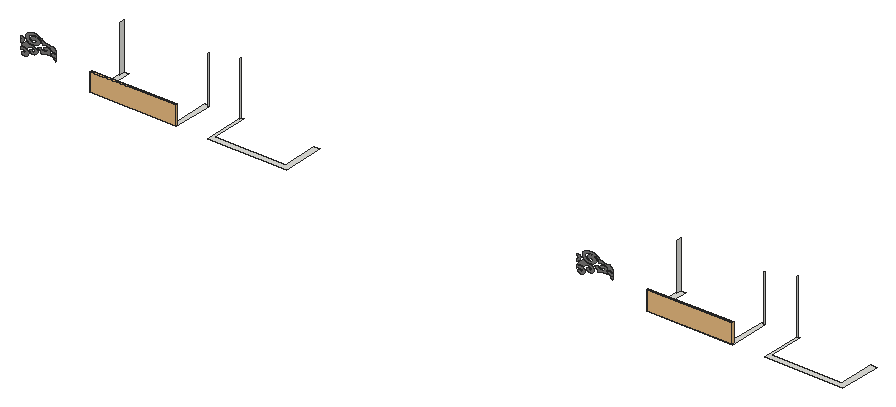
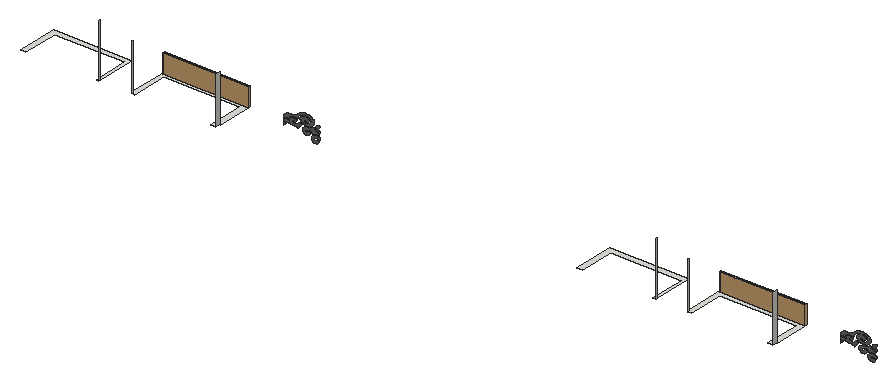
# SketchUp Ruby script. Lengths in inches.
U = 1.inch
M = Sketchup.active_model
def pt(a) = Geom::Point3d.new(a.map { |v| v * U })
def face(e, loops, mat)
  f = e.add_face(loops[0].map { |a| pt(a) })
  loops[1..].each { |l| e.add_face(l.map { |a| pt(a) }).erase! }
  f.material = f.back_material = mat if mat
  f
end
# faces: each face lists its corners as indices into pts; further lists are holes
def faces(e, pts, list, mat = nil) = list.each { |f| face(e, (f[0].is_a?(Array) ? f : [f]).map { |l| l.map { |i| pts[i] } }, mat) }
# xy, xz, yz: faces in a plane at the given z, y or x. An outline is a flat list of corners, or four numbers for a rectangle; further outlines are holes
def ring(l) = l.size == 4 ? [[l[0], l[1]], [l[2], l[1]], [l[2], l[3]], [l[0], l[3]]] : l.each_slice(2).to_a
def flat(e, list, mat, &to3) = list.each { |f| face(e, (f[0].is_a?(Array) ? f : [f]).map { |l| ring(l).map { |u, v| to3.(u, v) } }, mat) }
def xy(e, z, list, mat = nil) = flat(e, list, mat) { |x, y| [x, y, z] }
def xz(e, y, list, mat = nil) = flat(e, list, mat) { |x, z| [x, y, z] }
def yz(e, x, list, mat = nil) = flat(e, list, mat) { |y, z| [x, y, z] }
def lines(e, pts, list) = list.each { |a, b| e.add_line(pt(pts[a]), pt(pts[b])) }
# prism: a flat outline (further loops are holes) pulled along v
def prism(e, loops, v, mat = nil)
  f = face(e, loops, mat); d = Geom::Vector3d.new(v.map { |x| x * U })
  f.pushpull(f.normal.samedirection?(d) ? d.length : -d.length)
end
def box(e, o, s, mat = nil) = prism(e, [[o, [o[0] + s[0], o[1], o[2]], [o[0] + s[0], o[1] + s[1], o[2]], [o[0], o[1] + s[1], o[2]]]], [0, 0, s[2]], mat)
def at(x, y, z, deg = 0) = Geom::Transformation.translation(pt([x, y, z])) * Geom::Transformation.rotation(ORIGIN, Z_AXIS, deg.degrees)
def axes(o, x, y, z) = Geom::Transformation.new([*x, 0, *y, 0, *z, 0, *pt(o).to_a, 1])
def part(name) = M.definitions.add(name)
# library, detail: a bought-in or finely detailed component or shape, given as its bounding box
def library(name, o, s) = part(name).tap { |d| box(d.entities, o, s) }
def detail(e, o, s) = box(e.add_group.entities, o, s)
def put(e, d, t, mat = nil) = e.add_instance(d, t).tap { |i| i.material = mat if mat }
def group(e, t, mat = nil) = e.add_group.tap { |g| g.transformation = t; g.material = mat if mat }.entities
root = M.entities
M.materials.add("[0043_SaddleBrown]4").color = [124, 123, 122]
c1 = library("Glass Railing",[0,0,0],[139.5,4.76,42])
xy(root,541.1875,[[3051.26,558.125,3245.44,558.125,3245.44,647.91,3243.69,647.91,3243.69,651.03,3235.84,651.03,3235.84,570.83,3064.33,570.83,3064.33,651.03,3053.01,651.03,3053.01,640.11,3051.26,640.11],[3315.93,558.125,3493.19,558.125,3493.19,651.03,3480.11,651.03,3480.11,570.83,3322.22,570.83,3322.22,651.03,3315.93,651.03],[4301.88,558.125,4496.07,558.125,4496.07,647.91,4494.32,647.91,4494.32,651.03,4486.46,651.03,4486.46,570.83,4314.96,570.83,4314.96,651.03,4303.63,651.03,4303.63,640.11,4301.88,640.11],[4566.56,558.125,4743.81,558.125,4743.81,651.03,4730.74,651.03,4730.74,570.83,4572.84,570.83,4572.84,651.03,4566.56,651.03]])
xz(root,589.17,[[2879.79,541.67,2878.5,541.71,2877.26,541.9,2876.09,542.23,2875.05,542.69,2874.17,543.27,2873.48,543.93,2873,544.67,2872.76,545.44,2872.67,545.74,2872.68,546.04,2872.78,546.34,2872.97,546.62,2873.25,546.875,2873.6,547.09,2874.02,547.26,2874.48,547.37,2874.96,547.43,2875.46,547.43,2875.94,547.37,2876.4,547.25,2876.67,547.03,2876.96,546.83,2877.27,546.64,2877.59,546.45,2877.94,546.29,2878.3,546.13,2878.68,545.99,2879.07,545.87,2879.48,545.76,2879.89,545.66,2880.3125,545.58,2880.74,545.52,2881.31,545.82,2881.8,546.16,2882.23,546.53,2882.58,546.93,2882.85,547.36,2883.03,547.8,2883.13,548.25,2883.13,548.71,2883.04,549.16,2882.86,549.6,2882.6,550.03,2882.25,550.43,2881.52,551.04,2880.63,551.56,2879.62,551.98,2878.5,552.29,2877.3125,552.48,2876.09,552.55,2874.87,552.48,2873.68,552.29,2872.5625,551.98,2871.55,551.56,2870.66,551.04,2869.93,550.43,2869.93,554.9,2870.81,555.28,2871.74,555.61,2872.72,555.89,2873.74,556.1,2874.79,556.26,2875.85,556.35,2876.93,556.37,2878,556.33,2879.07,556.23,2880.11,556.07,2881.12,555.84,2882.09,555.55,2883.79,554.88,2885.29,554.04,2886.55,553.07,2887.54,551.99,2888.24,550.82,2888.62,549.61,2888.68,548.36,2888.42,547.13,2887.84,545.94,2886.95,544.83,2885.79,543.8125,2884.375,542.92,2883.4,542.41,2882.28,542.02,2881.06,541.77],[4130.41,541.67,4129.13,541.71,4127.88,541.9,4126.72,542.23,4125.67,542.69,4124.79,543.27,4124.1,543.93,4123.625,544.67,4123.39,545.44,4123.3,545.74,4123.3,546.04,4123.4,546.34,4123.6,546.62,4123.875,546.875,4124.23,547.09,4124.64,547.26,4125.1,547.37,4125.59,547.43,4126.08,547.43,4126.57,547.37,4127.03,547.25,4127.29,547.03,4127.58,546.83,4127.89,546.64,4128.22,546.45,4128.57,546.29,4128.93,546.13,4129.31,545.99,4129.7,545.87,4130.1,545.76,4130.51,545.66,4130.9375,545.58,4131.37,545.52,4131.93,545.82,4132.43,546.16,4132.86,546.53,4133.21,546.93,4133.48,547.36,4133.66,547.8,4133.75,548.25,4133.75,548.71,4133.66,549.16,4133.49,549.6,4133.22,550.03,4132.87,550.43,4132.14,551.04,4131.26,551.56,4130.24,551.98,4129.125,552.29,4127.9375,552.48,4126.71,552.55,4125.49,552.48,4124.3,552.29,4123.1875,551.98,4122.17,551.56,4121.29,551.04,4120.56,550.43,4120.56,554.9,4121.43,555.28,4122.36,555.61,4123.34,555.89,4124.36,556.1,4125.41,556.26,4126.48,556.35,4127.55,556.37,4128.63,556.33,4129.69,556.23,4130.74,556.07,4131.75,555.84,4132.72,555.55,4134.41,554.88,4135.91,554.04,4137.17,553.07,4138.16,551.99,4138.86,550.82,4139.24,549.61,4139.31,548.36,4139.04,547.13,4138.46,545.94,4137.58,544.83,4136.41,543.8125,4135,542.92,4134.02,542.41,4132.9,542.02,4131.68,541.77],[2899.8,551.33,2898.2,551.39,2896.65,551.65,2895.22,552.1,2893.98,552.73,2892.98,553.5,2892.27,554.38,2891.87,555.34,2891.8125,556.33,2891.875,556.63,2891.99,556.93,2892.15,557.23,2892.36,557.51,2892.62,557.77,2892.92,558.02,2893.25,558.25,2893.63,558.46,2894.04,558.64,2894.48,558.79,2894.94,558.92,2895.41,559.01,2895.5,558.58,2895.62,558.15,2895.78,557.72,2895.99,557.3,2896.23,556.89,2896.51,556.49,2896.83,556.1,2897.18,555.72,2897.58,555.35,2898,555,2898.46,554.67,2898.95,554.35,2899.88,554.64,2900.73,555.01,2901.48,555.46,2902.11,555.97,2902.6,556.54,2902.9375,557.15,2903.125,557.78,2903.15,558.42,2903.01,559.06,2902.72,559.68,2902.27,560.26,2901.6875,560.79,2900.85,561.59,2899.78,562.28,2898.53,562.84,2897.125,563.25,2895.62,563.49,2894.07,563.5625,2892.53,563.45,2891.05,563.17,2889.68,562.72,2888.46,562.13,2887.45,561.41,2886.67,560.59,2886.45,560.37,2886.25,560.14,2886.06,559.91,2885.88,559.68,2885.71,559.45,2885.56,559.21,2885.42,558.97,2885.29,558.72,2885.17,558.47,2885.07,558.23,2884.98,557.97,2884.91,557.72,2884.22,558.29,2883.41,558.79,2882.52,559.24,2881.54,559.61,2880.49,559.9,2879.39,560.11,2878.26,560.23,2877.11,560.27,2875.97,560.22,2874.84,560.08,2873.75,559.86,2872.71,559.56,2872.92,559.82,2873.12,560.09,2873.28,560.37,2873.42,560.65,2873.54,560.94,2873.62,561.23,2873.68,561.53,2873.71,561.82,2873.72,562.12,2873.69,562.41,2873.64,562.71,2873.5625,563,2874.7,563.53,2875.8,564.1,2876.86,564.7,2877.86,565.33,2878.81,565.99,2879.72,566.67,2880.5625,567.39,2881.36,568.12,2882.09,568.88,2882.76,569.66,2883.37,570.46,2883.92,571.27,2884.53,570.61,2885.24,569.98,2886.0625,569.4,2886.97,568.88,2887.96,568.41,2889.02,568.01,2890.14,567.68,2891.3125,567.42,2892.52,567.24,2893.76,567.13,2895,567.1,2896.24,567.14,2898.66,566.8,2900.95,566.2,2903.02,565.37,2904.83,564.32,2906.32,563.1,2907.4375,561.74,2908.15,560.28,2908.4375,558.77,2908.29,557.24,2907.71,555.76,2906.73,554.36,2905.36,553.09,2904.23,552.39,2902.89,551.85,2901.39,551.49],[4150.43,551.33,4148.82,551.39,4147.27,551.65,4145.84,552.1,4144.6,552.73,4143.6,553.5,4142.89,554.38,4142.5,555.34,4142.4375,556.33,4142.5,556.63,4142.61,556.93,4142.77,557.23,4142.98,557.51,4143.24,557.77,4143.54,558.02,4143.88,558.25,4144.26,558.46,4144.66,558.64,4145.1,558.79,4145.56,558.92,4146.04,559.01,4146.12,558.58,4146.24,558.15,4146.41,557.72,4146.61,557.3,4146.85,556.89,4147.14,556.49,4147.45,556.1,4147.81,555.72,4148.2,555.35,4148.625,555,4149.08,554.67,4149.57,554.35,4150.51,554.64,4151.36,555.01,4152.11,555.46,4152.73,555.97,4153.22,556.54,4153.5625,557.15,4153.75,557.78,4153.77,558.42,4153.64,559.06,4153.34,559.68,4152.9,560.26,4152.3125,560.79,4151.47,561.59,4150.41,562.28,4149.15,562.84,4147.75,563.25,4146.25,563.49,4144.7,563.5625,4143.16,563.45,4141.68,563.17,4140.3,562.72,4139.09,562.13,4138.07,561.41,4137.29,560.59,4137.08,560.37,4136.87,560.14,4136.68,559.91,4136.5,559.68,4136.34,559.45,4136.18,559.21,4136.04,558.97,4135.91,558.72,4135.8,558.47,4135.7,558.23,4135.61,557.97,4135.53,557.72,4134.84,558.29,4134.04,558.79,4133.14,559.24,4132.16,559.61,4131.12,559.9,4130.02,560.11,4128.89,560.23,4127.74,560.27,4126.59,560.22,4125.46,560.08,4124.37,559.86,4123.33,559.56,4123.55,559.82,4123.74,560.09,4123.91,560.37,4124.05,560.65,4124.16,560.94,4124.25,561.23,4124.31,561.53,4124.34,561.82,4124.34,562.12,4124.32,562.41,4124.27,562.71,4124.1875,563,4125.33,563.53,4126.43,564.1,4127.48,564.7,4128.49,565.33,4129.44,565.99,4130.34,566.67,4131.1875,567.39,4131.98,568.12,4132.71,568.88,4133.39,569.66,4134,570.46,4134.54,571.27,4135.15,570.61,4135.87,569.98,4136.6875,569.4,4137.59,568.88,4138.58,568.41,4139.65,568.01,4140.77,567.68,4141.9375,567.42,4143.15,567.24,4144.38,567.13,4145.625,567.1,4146.87,567.14,4149.29,566.8,4151.57,566.2,4153.65,565.37,4155.46,564.32,4156.94,563.1,4158.0625,561.74,4158.77,560.28,4159.0625,558.77,4158.92,557.24,4158.34,555.76,4157.35,554.36,4155.98,553.09,4154.85,552.39,4153.51,551.85,4152.01,551.49],[2950.32,553.96,2950.04,554.34,2949.75,554.71,2949.45,555.08,2949.13,555.4375,2948.8,555.8,2948.46,556.15,2948.11,556.5,2947.75,556.85,2947.37,557.19,2946.98,557.53,2946.59,557.86,2946.18,558.1875,2946.45,558.35,2946.75,558.5,2947.06,558.64,2947.38,558.76,2947.72,558.86,2948.08,558.95,2948.4375,559.03,2948.81,559.09,2949.18,559.13,2949.5625,559.15,2949.94,559.16,2950.32,559.15],
  [4200.95,553.96,4200.67,554.34,4200.375,554.71,4200.07,555.08,4199.76,555.4375,4199.43,555.8,4199.09,556.15,4198.37,556.85,4198,557.19,4197.61,557.53,4197.21,557.86,4196.8,558.1875,4197.08,558.35,4197.37,558.5,4197.68,558.64,4198.01,558.76,4198.35,558.86,4198.7,558.95,4199.0625,559.03,4199.43,559.09,4199.81,559.13,4200.1875,559.15,4200.57,559.16,4200.95,559.15],[2917.28,558.48,2917.16,559.39,2916.93,560.29,2916.59,561.18,2916.15,562.05,2915.6,562.9,2914.94,563.72,2914.19,564.51,2913.35,565.26,2912.41,565.97,2911.4,566.63,2910.3,567.25,2909.13,567.8125,2909.75,567.99,2910.36,568.17,2910.97,568.36,2911.57,568.55,2912.75,568.97,2913.33,569.18,2913.9,569.41,2914.46,569.64,2915.02,569.88,2915.57,570.125,2916.11,570.38,2916.21,569.18,2916.74,568.03,2917.66,566.98,2918.93,566.07,2920.5,565.36,2922.27,564.87,2924.18,564.625,2926.13,564.65,2928.02,564.93,2929.77,565.45,2931.3,566.2,2932.52,567.13,2932.55,567.42,2932.57,567.71,2932.58,568,2932.57,568.29,2932.55,568.58,2932.51,568.87,2932.46,569.16,2932.4,569.45,2932.32,569.73,2932.23,570.02,2932.12,570.3,2932,570.58,2931.41,570.74,2930.78,570.84,2930.13,570.875,2929.49,570.85,2928.86,570.76,2928.26,570.61,2927.7,570.4,2927.21,570.14,2926.79,569.84,2926.45,569.5,2926.21,569.13,2926.07,568.74,2925.66,568.85,2925.27,568.97,2924.89,569.11,2924.52,569.26,2924.18,569.43,2923.84,569.61,2923.53,569.8,2923.24,570,2922.97,570.22,2922.72,570.44,2922.5,570.68,2922.3,570.92,2922.89,571.87,2923.78,572.73,2924.9375,573.46,2926.3125,574.03,2927.85,574.42,2929.49,574.6,2931.15,574.58,2932.76,574.35,2934.27,573.91,2935.6,573.3,2936.7,572.54,2937.52,571.65,2936.96,570.85,2936.51,570.02,2936.1875,569.17,2935.99,568.3125,2935.91,567.44,2935.96,566.57,2936.14,565.7,2936.4375,564.85,2936.86,564.02,2937.4,563.21,2938.06,562.4375,2938.82,561.7,2936.94,561.8,2935.06,561.83,2933.17,561.79,2931.29,561.68,2929.43,561.51,2927.59,561.27,2925.77,560.96,2923.98,560.59,2922.23,560.15,2920.53,559.66,2918.88,559.1],[4167.91,558.48,4167.79,559.39,4167.56,560.29,4167.22,561.18,4166.77,562.05,4166.22,562.9,4165.57,563.72,4164.82,564.51,4163.97,565.26,4163.04,565.97,4162.02,566.63,4160.92,567.25,4159.76,567.8125,4160.375,567.99,4160.99,568.17,4162.19,568.55,4163.37,568.97,4163.95,569.18,4165.09,569.64,4165.64,569.88,4166.19,570.125,4166.73,570.38,4166.84,569.18,4167.36,568.03,4168.29,566.98,4169.56,566.07,4171.12,565.36,4172.9,564.87,4174.81,564.625,4176.75,564.65,4178.65,564.93,4180.4,565.45,4181.92,566.2,4183.14,567.13,4183.18,567.42,4183.2,567.71,4183.21,568,4183.2,568.29,4183.18,568.58,4183.14,568.87,4183.09,569.16,4183.03,569.45,4182.95,569.73,4182.85,570.02,4182.75,570.3,4182.63,570.58,4182.03,570.74,4181.41,570.84,4180.76,570.875,4180.11,570.85,4179.48,570.76,4178.88,570.61,4178.33,570.4,4177.84,570.14,4177.42,569.84,4177.08,569.5,4176.84,569.13,4176.69,568.74,4176.29,568.85,4175.89,568.97,4175.51,569.11,4175.15,569.26,4174.8,569.43,4174.47,569.61,4174.16,569.8,4173.87,570,4173.6,570.22,4173.35,570.44,4173.125,570.68,4172.92,570.92,4173.51,571.87,4174.4,572.73,4175.5625,573.46,4176.9375,574.03,4178.48,574.42,4180.11,574.6,4181.77,574.58,4183.39,574.35,4184.89,573.91,4186.23,573.3,4187.32,572.54,4188.15,571.65,4187.58,570.85,4187.14,570.02,4186.8125,569.17,4186.61,568.3125,4186.54,567.44,4186.59,566.57,4186.76,565.7,4187.0625,564.85,4187.49,564.02,4188.03,563.21,4188.68,562.4375,4189.45,561.7,4187.57,561.8,4185.68,561.83,4183.8,561.79,4181.92,561.68,4180.06,561.51,4178.21,561.27,4176.39,560.96,4174.61,560.59,4172.86,560.15,4171.16,559.66,4169.5,559.1],[2946.1,561.42,2945.01,561.51,2943.94,561.71,2942.95,562.01,2942.04,562.41,2941.25,562.89,2940.6,563.4375,2940.09,564.04,2939.75,564.69,2939.49,564.99,2939.33,565.31,2939.28,565.64,2939.33,565.97,2939.48,566.29,2939.74,566.59,2940.07,566.85,2940.49,567.07,2940.97,567.23,2941.48,567.33,2942.02,567.375,2942.57,567.35,2943.03,567.29,2943.48,567.21,2943.92,567.1,2944.34,566.96,2944.74,566.81,2945.12,566.63,2945.46,566.43,2945.78,566.22,2946.07,565.98,2946.32,565.74,2946.54,565.48,2946.71,565.21,2947.06,565.32,2947.4,565.45,2947.73,565.58,2948.05,565.71,2948.37,565.86,2948.97,566.16,2949.26,566.33,2949.54,566.5,2949.8125,566.67,2950.07,566.85,2950.32,567.04,2950.32,562.11,2949.35,561.78,2948.3,561.56,2947.21,561.43],[4196.73,561.42,4195.63,561.51,4194.57,561.71,4193.57,562.01,4192.67,562.41,4191.88,562.89,4191.22,563.4375,4190.71,564.04,4190.37,564.69,4190.12,564.99,4189.96,565.31,4189.9,565.64,4189.95,565.97,4190.11,566.29,4190.36,566.59,4190.7,566.85,4191.12,567.07,4191.59,567.23,4192.11,567.33,4192.65,567.375,4193.19,567.35,4193.66,567.29,4194.11,567.21,4194.55,567.1,4194.97,566.96,4195.37,566.81,4195.74,566.63,4196.09,566.43,4196.41,566.22,4196.69,565.98,4196.95,565.74,4197.16,565.48,4197.34,565.21,4197.68,565.32,4198.02,565.45,4198.68,565.71,4199.3,566.01,4199.6,566.16,4199.89,566.33,4200.17,566.5,4200.4375,566.67,4200.7,566.85,4200.95,567.04,4200.95,562.11,4199.97,561.78,4198.93,561.56,4197.84,561.43],
  [2869.93,564.47,2869.93,568.51,2871.02,568.79,2871.98,569.2,2872.78,569.74,2873.38,570.36,2873.75,571.04,2873.875,571.76,2873.75,572.48,2873.38,573.17,2872.78,573.79,2871.98,574.32,2871.02,574.73,2869.93,575.01,2869.93,578.44,2871.18,578.38,2872.4,578.2,2873.5625,577.92,2874.64,577.52,2875.61,577.03,2876.44,576.46,2877.125,575.8125,2877.64,575.11,2877.98,574.37,2878.13,573.61,2878.1,572.84,2877.87,572.08,2877.52,571.34,2877.11,570.62,2876.64,569.91,2876.1,569.22,2875.52,568.55,2874.87,567.89,2874.17,567.26,2873.42,566.65,2872.62,566.0625,2871.77,565.5,2870.87,564.97],[4120.56,564.47,4120.56,568.51,4121.64,568.79,4122.61,569.2,4123.4,569.74,4124,570.36,4124.375,571.04,4124.5,571.76,4124.375,572.48,4124,573.17,4123.4,573.79,4122.61,574.32,4121.64,574.73,4120.56,575.01,4120.56,578.44,4121.81,578.38,4123.03,578.2,4124.1875,577.92,4125.26,577.52,4126.23,577.03,4127.07,576.46,4127.75,575.8125,4128.27,575.11,4128.61,574.37,4128.76,573.61,4128.72,572.84,4128.49,572.08,4128.14,571.34,4127.73,570.62,4127.26,569.91,4126.73,569.22,4126.14,568.55,4125.5,567.89,4124.8,567.26,4124.05,566.65,4123.24,566.0625,4122.39,565.5,4121.5,564.97],[2950.32,568.52,2949.96,569.11,2949.46,569.67,2948.84,570.17,2948.11,570.62,2947.29,571,2946.38,571.3125,2945.42,571.54,2944.41,571.68,2943.38,571.73,2942.35,571.69,2941.34,571.57,2940.37,571.36,2939.92,572.72,2939.11,574.02,2937.94,575.22,2936.47,576.27,2934.72,577.15,2932.75,577.84,2930.62,578.31,2928.38,578.55,2926.12,578.55,2923.89,578.32,2921.75,577.85,2919.78,577.17,2919.72,578.89,2919.25,580.59,2918.39,582.23,2917.14,583.77,2915.55,585.19,2913.64,586.45,2911.45,587.53,2909.04,588.4,2906.4375,589.05,2903.71,589.45,2900.92,589.61,2898.12,589.52,2895.67,588.91,2893.45,588.01,2891.56,586.87,2890.07,585.52,2889.02,584.03,2888.47,582.4375,2888.43,580.81,2888.89,579.21,2889.86,577.6875,2891.28,576.31,2893.11,575.14,2895.27,574.19,2896.66,573.82,2898.16,573.62,2899.68,573.61,2901.18,573.8,2902.58,574.17,2903.83,574.7,2904.875,575.38,2905.67,576.18,2906.1875,577.0625,2906.4,577.99,2906.3,578.93,2905.9,579.83,2905.62,580.16,2905.24,580.45,2904.78,580.69,2904.25,580.87,2903.67,580.98,2903.06,581.02,2902.46,580.98,2901.88,580.87,2901.35,580.69,2900.89,580.45,2900.51,580.16,2900.23,579.83,2900.09,579.64,2899.93,579.45,2899.75,579.28,2899.54,579.11,2899.31,578.95,2899.06,578.8125,2898.79,578.68,2898.5,578.57,2898.2,578.46,2897.89,578.38,2897.57,578.31,2897.24,578.25,2896.66,578.46,2896.125,578.72,2895.64,579.01,2895.22,579.33,2894.87,579.69,2894.59,580.0625,2894.39,580.46,2894.27,580.87,2894.23,581.28,2894.27,581.69,2894.4,582.1,2894.61,582.49,2895,583.02,2895.48,583.52,2896.04,583.99,2896.68,584.42,2897.4,584.8,2898.17,585.13,2899,585.41,2899.88,585.63,2900.79,585.8,2901.72,585.9,2902.66,585.94,2903.61,585.92,2905.1,585.78,2906.55,585.51,2907.92,585.13,2909.2,584.64,2910.37,584.05,2911.39,583.36,2912.26,582.6,2912.95,581.78,2913.46,580.91,2913.78,580,2913.9,579.08,2913.81,578.15,2913.2,576.76,2912.28,575.43,2911.0625,574.2,2909.57,573.09,2907.84,572.12,2905.89,571.31,2903.79,570.67,2901.55,570.23,2899.24,569.99,2896.89,569.95,2894.5625,570.11,2892.29,570.48,2890.1,571.41,2888.12,572.5,2886.38,573.73,2884.92,575.1,2883.76,576.57,2882.92,578.12,2882.42,579.73,2882.26,581.36,2882.4375,582.99,2882.96,584.59,2883.82,586.14,2884.99,587.6,2886.8,589.2,2889.02,590.58,2891.59,591.72,2894.43,592.57,2897.46,593.12,2900.61,593.34,2903.77,593.23,2906.85,592.8,2909.77,592.05,2912.44,591.01,2914.79,589.71,2916.75,588.1875,2917.29,587.55,2917.88,586.9375,2918.52,586.34,2919.2,585.76,2919.92,585.2,2920.69,584.66,2921.5,584.14,2922.35,583.65,2923.23,583.1875,2924.15,582.75,2925.1,582.33,2926.08,581.95,2927.38,581.57,2928.72,581.23,2930.08,580.94,2931.47,580.7,2932.875,580.5,2934.3,580.36,2935.73,580.26,2937.17,580.2,2938.61,580.2,2940.05,580.25,2941.48,580.34,2942.91,580.49,2943.46,579.94,2944.03,579.4,2944.61,578.86,2945.2,578.33,2945.8,577.81,2946.42,577.28,2947.04,576.77,2948.32,575.75,2948.98,575.25,2949.65,574.75,2950.32,574.26],[4200.95,568.52,4200.58,569.11,4200.08,569.67,4199.46,570.17,4198.74,570.62,4197.91,571,4197.01,571.3125,4196.04,571.54,4195.04,571.68,4194.01,571.73,4192.98,571.69,4191.97,571.57,4190.99,571.36,4190.55,572.72,4189.73,574.02,4188.57,575.22,4187.09,576.27,4185.34,577.15,4183.37,577.84,4181.24,578.31,4179.01,578.55,4176.74,578.55,4174.51,578.32,4172.38,577.85,4170.4,577.17,4170.34,578.89,4169.875,580.59,4169.01,582.23,4167.77,583.77,4166.18,585.19,4164.27,586.45,4162.08,587.53,4159.66,588.4,4157.0625,589.05,4154.34,589.45,4151.55,589.61,4148.75,589.52,4146.29,588.91,4144.08,588.01,4142.19,586.87,4140.69,585.52,4139.65,584.03,4139.09,582.4375,4139.05,580.81,4139.52,579.21,4140.48,577.6875,4141.9,576.31,4143.73,575.14,4145.89,574.19,4147.29,573.82,4148.78,573.62,4150.31,573.61,4151.8,573.8,4153.2,574.17,4154.45,574.7,4155.5,575.38,4156.3,576.18,4156.8125,577.0625,4157.03,577.99,4156.93,578.93,4156.52,579.83,4156.25,580.16,4155.87,580.45,4155.4,580.69,4154.87,580.87,4154.29,580.98,4153.69,581.02,4153.09,580.98,4152.51,580.87,4151.97,580.69,4151.51,580.45,4151.13,580.16,4150.86,579.83,4150.72,579.64,4150.56,579.45,4150.37,579.28,4150.16,579.11,4149.93,578.95,4149.68,578.8125,4149.41,578.68,4149.13,578.57,4148.83,578.46,4148.52,578.38,4148.19,578.31,4147.86,578.25,4147.28,578.46,4146.75,578.72,4146.27,579.01,4145.85,579.33,4145.5,579.69,4145.22,580.0625,4145.02,580.46,4144.9,580.87,4144.86,581.28,4144.9,581.69,4145.03,582.1,4145.23,582.49,4145.62,583.02,4146.1,583.52,4146.67,583.99,4147.31,584.42,4148.02,584.8,4148.8,585.13,4149.63,585.41,4150.5,585.63,4151.41,585.8,4152.34,585.9,4153.29,585.94,4154.23,585.92,4155.72,585.78,4157.17,585.51,4158.55,585.13,4159.83,584.64,4160.99,584.05,4162.02,583.36,4162.88,582.6,4163.58,581.78,4164.09,580.91,4164.4,580,4164.52,579.08,4164.43,578.15,4163.83,576.76,4162.91,575.43,4161.6875,574.2,4160.19,573.09,4158.46,572.12,4156.52,571.31,4154.41,570.67,4152.18,570.23,4149.86,569.99,4147.52,569.95,4145.1875,570.11,4142.92,570.48,4140.72,571.41,4138.74,572.5,4137.01,573.73,4135.55,575.1,4134.39,576.57,4133.55,578.12,4133.04,579.73,4132.88,581.36,4133.0625,582.99,4133.59,584.59,4134.44,586.14,4135.62,587.6,4137.42,589.2,4139.64,590.58,4142.21,591.72,4145.05,592.57,4148.09,593.12,4151.23,593.34,4154.39,593.23,4157.47,592.8,4160.39,592.05,4163.07,591.01,4165.42,589.71,4167.375,588.1875,4167.92,587.55,4168.51,586.9375,4169.14,586.34,4169.82,585.76,4170.55,585.2,4171.32,584.66,4172.125,584.14,4172.97,583.65,4173.85,583.1875,4174.77,582.75,4175.72,582.33,4176.71,581.95,4178.01,581.57,4179.34,581.23,4180.71,580.94,4182.09,580.7,4183.5,580.5,4184.92,580.36,4186.35,580.26,4187.79,580.2,4189.24,580.2,4190.68,580.25,4192.11,580.34,4193.53,580.49,4194.09,579.94,4194.66,579.4,4195.24,578.86,4195.83,578.33,4196.43,577.81,4197.04,577.28,4198.3,576.26,4198.95,575.75,4199.6,575.25,4200.27,574.75,4200.95,574.26]],"[0043_SaddleBrown]4")
xz(root,651.03,[[3315.93,541.1875,3316.14,662.4375],[4566.56,541.1875,4566.77,662.4375]])
yz(root,3053.01,[[640.11,541.1875,651.03,646.4375]])
yz(root,3243.69,[[647.91,541.1875,651.03,646.4375]])
yz(root,3315.93,[[648.85,541.1875,651.03,662.4375]])
yz(root,4303.63,[[640.11,541.1875,651.03,646.4375]])
yz(root,4494.32,[[647.91,541.1875,651.03,646.4375]])
yz(root,4566.56,[[648.85,541.1875,651.03,662.4375]])
p = [[2933.23,589.17,546.54],[2933.14,589.17,547],[4183.85,589.17,546.54],[4183.77,589.17,547]]
lines(root,p,[[0,1],[2,3]])
put(root,c1,axes([3051.26,558.125,541.1875],[1.37946,0,0],[0,1,0],[0,0,1]))
put(root,c1,axes([4301.88,558.125,541.1875],[1.37946,0,0],[0,1,0],[0,0,1]))
